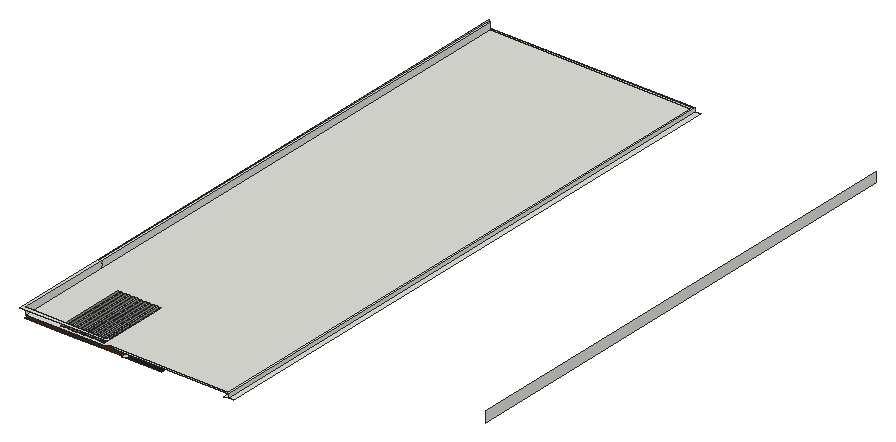
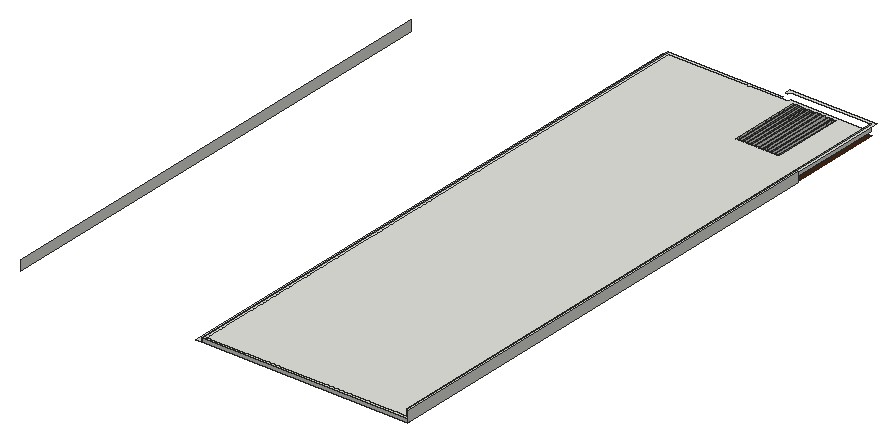
# SketchUp Ruby script. Lengths in inches.
U = 1.inch
M = Sketchup.active_model
def pt(a) = Geom::Point3d.new(a.map { |v| v * U })
def face(e, loops, mat)
  f = e.add_face(loops[0].map { |a| pt(a) })
  loops[1..].each { |l| e.add_face(l.map { |a| pt(a) }).erase! }
  f.material = f.back_material = mat if mat
  f
end
# faces: each face lists its corners as indices into pts; further lists are holes
def faces(e, pts, list, mat = nil) = list.each { |f| face(e, (f[0].is_a?(Array) ? f : [f]).map { |l| l.map { |i| pts[i] } }, mat) }
# xy, xz, yz: faces in a plane at the given z, y or x. An outline is a flat list of corners, or four numbers for a rectangle; further outlines are holes
def ring(l) = l.size == 4 ? [[l[0], l[1]], [l[2], l[1]], [l[2], l[3]], [l[0], l[3]]] : l.each_slice(2).to_a
def flat(e, list, mat, &to3) = list.each { |f| face(e, (f[0].is_a?(Array) ? f : [f]).map { |l| ring(l).map { |u, v| to3.(u, v) } }, mat) }
def xy(e, z, list, mat = nil) = flat(e, list, mat) { |x, y| [x, y, z] }
def xz(e, y, list, mat = nil) = flat(e, list, mat) { |x, z| [x, y, z] }
def yz(e, x, list, mat = nil) = flat(e, list, mat) { |y, z| [x, y, z] }
def lines(e, pts, list) = list.each { |a, b| e.add_line(pt(pts[a]), pt(pts[b])) }
# prism: a flat outline (further loops are holes) pulled along v
def prism(e, loops, v, mat = nil)
  f = face(e, loops, mat); d = Geom::Vector3d.new(v.map { |x| x * U })
  f.pushpull(f.normal.samedirection?(d) ? d.length : -d.length)
end
def box(e, o, s, mat = nil) = prism(e, [[o, [o[0] + s[0], o[1], o[2]], [o[0] + s[0], o[1] + s[1], o[2]], [o[0], o[1] + s[1], o[2]]]], [0, 0, s[2]], mat)
def at(x, y, z, deg = 0) = Geom::Transformation.translation(pt([x, y, z])) * Geom::Transformation.rotation(ORIGIN, Z_AXIS, deg.degrees)
def axes(o, x, y, z) = Geom::Transformation.new([*x, 0, *y, 0, *z, 0, *pt(o).to_a, 1])
def part(name) = M.definitions.add(name)
# library, detail: a bought-in or finely detailed component or shape, given as its bounding box
def library(name, o, s) = part(name).tap { |d| box(d.entities, o, s) }
def detail(e, o, s) = box(e.add_group.entities, o, s)
def put(e, d, t, mat = nil) = e.add_instance(d, t).tap { |i| i.material = mat if mat }
def group(e, t, mat = nil) = e.add_group.tap { |g| g.transformation = t; g.material = mat if mat }.entities
root = M.entities
M.materials.add("[Color M08]").color = [30, 30, 30]
M.materials.add("[Field Square Tile]").color = [211, 167, 108]
M.materials.add("[Granite Light Gray]").color = [149, 148, 144]
M.materials.add("[Wood Veneer 01]").color = [66, 38, 20]
xy(root,380.5,[[2434.04,511.08,2434.04,1825.82,1986.28,1825.82,1986.28,762.17,2202.28,762.17,2202.28,727.2,1976.47,727.2,1976.47,1835.625,2443.85,1835.625,2443.85,511.08],[2202.28,511.08,2211.2,589.83],[2443.85,511.08,2455.66,1835.625],[2202.28,589.83,2202.28,762.17,1986.28,762.17,1986.28,1825.82,2434.04,1825.82,2434.04,589.83,2387.27,589.83,2387.27,697.21,2291.96,697.21,2291.96,738.02,2211.2,738.02,2211.2,697.21,2202.58,697.21,2202.58,589.83],[2202.58,589.83,2211.2,697.21],
  [2291.96,589.83,2387.27,697.21],[2211.2,697.21,2291.96,738.02]])
xy(root,380.5,[[2211.2,511.08,2291.96,697.21]],"[Color M08]")
xy(root,380.5,[[[1981.3,512.27,2053.23,727.2],[1998.33,606.01,1999.85,606.38,2001.23,607.14,2002.36,608.22,2003.17,609.56,2003.6,611.0625,2003.64,612.63,2003.26,614.15,2002.51,615.52,2001.42,616.65,2000.08,617.46,1998.58,617.9,1997.01,617.93,1995.49,617.56,1994.12,616.81,1992.99,615.72,1992.18,614.38,1991.74,612.875,1991.71,611.3125,1992.08,609.79,1992.84,608.42,1993.92,607.29,1995.26,606.48,1996.77,606.04],[2038.08,606.01,2039.6,606.38,2040.98,607.14,2042.11,608.22,2042.92,609.56,2043.35,611.0625,2043.39,612.63,2043.01,614.15,2042.26,615.52,2041.17,616.65,2039.83,617.46,2038.33,617.9,2036.76,617.93,2035.24,617.56,2033.87,616.81,2032.74,615.72,2031.93,614.38,2031.49,612.875,2031.46,611.3125,2031.83,609.79,2032.59,608.42,2033.67,607.29,2035.01,606.48,2036.52,606.04],[1998.33,554.26,1999.85,554.63,2001.23,555.39,2002.36,556.47,2003.17,557.81,2003.6,559.3125,2003.64,560.88,2003.26,562.4,2002.51,563.77,2001.42,564.9,2000.08,565.71,1998.58,566.15,1997.01,566.18,1995.49,565.81,1994.12,565.06,1992.99,563.97,1992.18,562.63,1991.74,561.125,1991.71,559.5625,1992.08,558.04,1992.84,556.67,1993.92,555.54,1995.26,554.73,1996.77,554.29],[2038.08,554.26,2039.6,554.63,2040.98,555.39,2042.11,556.47,2042.92,557.81,2043.35,559.3125,2043.39,560.88,2043.01,562.4,2042.26,563.77,2041.17,564.9,2039.83,565.71,2038.33,566.15,2036.76,566.18,2035.24,565.81,2033.87,565.06,2032.74,563.97,2031.93,562.63,2031.49,561.125,2031.46,559.5625,2031.83,558.04,2032.59,556.67,2033.67,555.54,2035.01,554.73,2036.52,554.29],[1998.33,523.51,1999.85,523.88,2001.23,524.64,2002.36,525.72,2003.17,527.06,2003.6,528.5625,2003.64,530.13,2003.26,531.65,2002.51,533.02,2001.42,534.15,2000.08,534.96,1998.58,535.4,1997.01,535.43,1995.49,535.06,1994.12,534.31,1992.99,533.22,1992.18,531.88,1991.74,530.375,1991.71,528.8125,1992.08,527.29,1992.84,525.92,1993.92,524.79,1995.26,523.98,1996.77,523.54],[2038.08,523.51,2039.6,523.88,2040.98,524.64,2042.11,525.72,2042.92,527.06,2043.35,528.5625,2043.39,530.13,2043.01,531.65,2042.26,533.02,2041.17,534.15,2039.83,534.96,2038.33,535.4,2036.76,535.43,2035.24,535.06,2033.87,534.31,2032.74,533.22,2031.93,531.88,2031.49,530.375,2031.46,528.8125,2031.83,527.29,2032.59,525.92,2033.67,524.79,2035.01,523.98,2036.52,523.54],[1998.33,666.01,1999.85,666.38,2001.23,667.14,2002.36,668.22,2003.17,669.56,2003.6,671.0625,2003.64,672.63,2003.26,674.15,2002.51,675.52,2001.42,676.65,2000.08,677.46,1998.58,677.9,1997.01,677.93,1995.49,677.56,1994.12,676.81,1992.99,675.72,1992.18,674.38,1991.74,672.875,1991.71,671.3125,1992.08,669.79,1992.84,668.42,1993.92,667.29,1995.26,666.48,1996.77,666.04],[2038.08,666.01,2039.6,666.38,2040.98,667.14,2042.11,668.22,2042.92,669.56,2043.35,671.0625,2043.39,672.63,2043.01,674.15,2042.26,675.52,2041.17,676.65,2039.83,677.46,2038.33,677.9,2036.76,677.93,2035.24,677.56,2033.87,676.81,2032.74,675.72,2031.93,674.38,2031.49,672.875,2031.46,671.3125,2031.83,669.79,2032.59,668.42,2033.67,667.29,2035.01,666.48,2036.52,666.04]],[[2053.23,512.27,2202.28,727.2],[2148.68,519.43,2154.93,680.49],[2139.56,519.43,2145.81,680.49],[2130.43,519.43,2136.68,680.49],[2121.31,519.43,2127.56,680.49],[2112.18,519.43,2118.43,680.49],[2103.06,519.43,2109.31,680.49],[2093.93,519.43,2100.18,680.49],[2084.81,519.43,2091.06,680.49],[2075.68,519.43,2081.93,680.49],[2066.56,519.43,2072.81,680.49],[2057.43,519.43,2063.68,680.49]]],"[Wood Veneer 01]")
xy(root,381.875,[[1998.33,554.26,1996.77,554.29,1995.26,554.73,1993.92,555.54,1992.84,556.67,1992.08,558.04,1991.71,559.5625,1991.74,561.125,1992.18,562.63,1992.99,563.97,1994.12,565.06,1995.49,565.81,1997.01,566.18,1998.58,566.15,2000.08,565.71,2001.42,564.9,2002.51,563.77,2003.26,562.4,2003.64,560.88,2003.6,559.3125,2003.17,557.81,2002.36,556.47,2001.23,555.39,1999.85,554.63],[2038.08,554.26,2036.52,554.29,2035.01,554.73,2033.67,555.54,2032.59,556.67,2031.83,558.04,2031.46,559.5625,2031.49,561.125,2031.93,562.63,2032.74,563.97,2033.87,565.06,2035.24,565.81,2036.76,566.18,2038.33,566.15,2039.83,565.71,2041.17,564.9,2042.26,563.77,2043.01,562.4,2043.39,560.88,2043.35,559.3125,2042.92,557.81,2042.11,556.47,2040.98,555.39,2039.6,554.63],[1998.33,606.01,1996.77,606.04,1995.26,606.48,1993.92,607.29,1992.84,608.42,1992.08,609.79,1991.71,611.3125,1991.74,612.875,1992.18,614.38,1992.99,615.72,1994.12,616.81,1995.49,617.56,1997.01,617.93,1998.58,617.9,2000.08,617.46,2001.42,616.65,2002.51,615.52,2003.26,614.15,2003.64,612.63,2003.6,611.0625,2003.17,609.56,2002.36,608.22,2001.23,607.14,1999.85,606.38],[2038.08,606.01,2036.52,606.04,2035.01,606.48,2033.67,607.29,2032.59,608.42,2031.83,609.79,2031.46,611.3125,2031.49,612.875,2031.93,614.38,2032.74,615.72,2033.87,616.81,2035.24,617.56,2036.76,617.93,2038.33,617.9,2039.83,617.46,2041.17,616.65,2042.26,615.52,2043.01,614.15,2043.39,612.63,2043.35,611.0625,2042.92,609.56,2042.11,608.22,2040.98,607.14,2039.6,606.38],[1998.33,666.01,1996.77,666.04,1995.26,666.48,1993.92,667.29,1992.84,668.42,1992.08,669.79,1991.71,671.3125,1991.74,672.875,1992.18,674.38,1992.99,675.72,1994.12,676.81,1995.49,677.56,1997.01,677.93,1998.58,677.9,2000.08,677.46,2001.42,676.65,2002.51,675.52,2003.26,674.15,2003.64,672.63,2003.6,671.0625,2003.17,669.56,2002.36,668.22,2001.23,667.14,1999.85,666.38],
  [2038.08,666.01,2036.52,666.04,2035.01,666.48,2033.67,667.29,2032.59,668.42,2031.83,669.79,2031.46,671.3125,2031.49,672.875,2031.93,674.38,2032.74,675.72,2033.87,676.81,2035.24,677.56,2036.76,677.93,2038.33,677.9,2039.83,677.46,2041.17,676.65,2042.26,675.52,2043.01,674.15,2043.39,672.63,2043.35,671.0625,2042.92,669.56,2042.11,668.22,2040.98,667.14,2039.6,666.38]],"[Field Square Tile]")
xy(root,388.625,[[[1982.81,510.87,2166.13,510.87,2166.13,517.43,2437.5,517.43,2437.5,1829.28,1982.81,1829.28],[2057.43,519.43,2063.68,680.49],[2066.56,519.43,2072.81,680.49],[2075.68,519.43,2081.93,680.49],[2084.81,519.43,2091.06,680.49],[2093.93,519.43,2100.18,680.49],[2103.06,519.43,2109.31,680.49],[2112.18,519.43,2118.43,680.49],[2121.31,519.43,2127.56,680.49],[2130.43,519.43,2136.68,680.49],[2139.56,519.43,2145.81,680.49],[2148.68,519.43,2154.93,680.49]],[2183.1875,511.08,2443.85,511.08,2443.85,1835.625,1976.47,1835.625,1982.81,1829.28,2437.5,1829.28,2437.5,517.43,2183.1875,517.43]])
xy(root,403.8125,[[1976.47,504.52,2172.48,504.52,2172.48,517.43,2166.13,517.43,2166.13,510.87,1982.81,510.87,1982.81,1829.28,1976.47,1835.625]])
xz(root,680.49,[[2057.43,380.5,2063.68,388.625],[2066.56,380.5,2072.81,388.625],[2075.68,380.5,2081.93,388.625],[2084.81,380.5,2091.06,388.625],[2093.93,380.5,2100.18,388.625],
  [2103.06,380.5,2109.31,388.625],[2112.18,380.5,2118.43,388.625],[2121.31,380.5,2127.56,388.625],[2130.43,380.5,2136.68,388.625],[2139.56,380.5,2145.81,388.625],
  [2148.68,380.5,2154.93,388.625]],"[Granite Light Gray]")
xz(root,1835.625,[[1976.47,380.5,2443.85,388.625]])
yz(root,1976.47,[[727.2,380.5,1835.625,403.8125]])
yz(root,1982.81,[[510.87,388.625,727.2,403.8125],[727.2,388.625,1829.28,403.8125]])
yz(root,2057.43,[[519.43,380.5,680.49,388.625]],"[Granite Light Gray]")
yz(root,2063.68,[[519.43,380.5,680.49,388.625]])
yz(root,2066.56,[[519.43,380.5,680.49,388.625]],"[Granite Light Gray]")
yz(root,2072.81,[[519.43,380.5,680.49,388.625]])
yz(root,2075.68,[[519.43,380.5,680.49,388.625]],"[Granite Light Gray]")
yz(root,2081.93,[[519.43,380.5,680.49,388.625]])
yz(root,2084.81,[[519.43,380.5,680.49,388.625]],"[Granite Light Gray]")
yz(root,2091.06,[[519.43,380.5,680.49,388.625]])
yz(root,2093.93,[[519.43,380.5,680.49,388.625]],"[Granite Light Gray]")
yz(root,2100.18,[[519.43,380.5,680.49,388.625]])
yz(root,2103.06,[[519.43,380.5,680.49,388.625]],"[Granite Light Gray]")
yz(root,2109.31,[[519.43,380.5,680.49,388.625]])
yz(root,2112.18,[[519.43,380.5,680.49,388.625]],"[Granite Light Gray]")
yz(root,2118.43,[[519.43,380.5,680.49,388.625]])
yz(root,2121.31,[[519.43,380.5,680.49,388.625]],"[Granite Light Gray]")
yz(root,2127.56,[[519.43,380.5,680.49,388.625]])
yz(root,2130.43,[[519.43,380.5,680.49,388.625]],"[Granite Light Gray]")
yz(root,2136.68,[[519.43,380.5,680.49,388.625]])
yz(root,2139.56,[[519.43,380.5,680.49,388.625]],"[Granite Light Gray]")
yz(root,2145.81,[[519.43,380.5,680.49,388.625]])
yz(root,2148.68,[[519.43,380.5,680.49,388.625]],"[Granite Light Gray]")
yz(root,2154.93,[[519.43,380.5,680.49,388.625]])
yz(root,2443.85,[[511.08,380.5,1835.625,388.625]])
yz(root,2855.22,[[727.2,380.5,1835.625,403.8125]])
p = [[1996.77,554.29,380.5],[1995.26,554.73,380.5],[1995.26,554.73,381.875],[1996.77,554.29,381.875],[1998.33,554.26,380.5],[1998.33,554.26,381.875],
  [1999.85,554.63,380.5],[1999.85,554.63,381.875],[2036.52,554.29,380.5],[2035.01,554.73,380.5],[2035.01,554.73,381.875],[2036.52,554.29,381.875],
  [2038.08,554.26,380.5],[2038.08,554.26,381.875],[2039.6,554.63,380.5],[2039.6,554.63,381.875],[2001.23,555.39,380.5],[2001.23,555.39,381.875],
  [2040.98,555.39,380.5],[2040.98,555.39,381.875],[1993.92,555.54,380.5],[1993.92,555.54,381.875],[2033.67,555.54,380.5],[2033.67,555.54,381.875],
  [2002.36,556.47,380.5],[2002.36,556.47,381.875],[2042.11,556.47,380.5],[2042.11,556.47,381.875],[1992.84,556.67,380.5],[1992.84,556.67,381.875],
  [2032.59,556.67,380.5],[2032.59,556.67,381.875],[2003.17,557.81,380.5],[2003.17,557.81,381.875],[2042.92,557.81,380.5],[2042.92,557.81,381.875],
  [1992.08,558.04,380.5],[1992.08,558.04,381.875],[2031.83,558.04,380.5],[2031.83,558.04,381.875],[2003.6,559.3125,380.5],[2003.6,559.3125,381.875],
  [2043.35,559.3125,380.5],[2043.35,559.3125,381.875],[1991.71,559.5625,380.5],[1991.71,559.5625,381.875],[2031.46,559.5625,380.5],[2031.46,559.5625,381.875],
  [2003.64,560.88,380.5],[2003.64,560.88,381.875],[2043.39,560.88,380.5],[2043.39,560.88,381.875],[1991.74,561.125,380.5],[1991.74,561.125,381.875],
  [2031.49,561.125,380.5],[2031.49,561.125,381.875],[2003.26,562.4,380.5],[2003.26,562.4,381.875],[2043.01,562.4,380.5],[2043.01,562.4,381.875],
  [1992.18,562.63,380.5],[1992.18,562.63,381.875],[2031.93,562.63,380.5],[2031.93,562.63,381.875],[2002.51,563.77,380.5],[2002.51,563.77,381.875],
  [2042.26,563.77,380.5],[2042.26,563.77,381.875],[1992.99,563.97,380.5],[1992.99,563.97,381.875],[2032.74,563.97,380.5],[2032.74,563.97,381.875],
  [2001.42,564.9,380.5],[2001.42,564.9,381.875],[2041.17,564.9,380.5],[2041.17,564.9,381.875],[1994.12,565.06,380.5],[1994.12,565.06,381.875],
  [2033.87,565.06,380.5],[2033.87,565.06,381.875],[2000.08,565.71,380.5],[2000.08,565.71,381.875],[2039.83,565.71,380.5],[2039.83,565.71,381.875],
  [1995.49,565.81,380.5],[1995.49,565.81,381.875],[2035.24,565.81,380.5],[2035.24,565.81,381.875],[1998.58,566.15,380.5],[1998.58,566.15,381.875],
  [2038.33,566.15,380.5],[2038.33,566.15,381.875],[1997.01,566.18,380.5],[1997.01,566.18,381.875],[2036.76,566.18,380.5],[2036.76,566.18,381.875],
  [1996.77,606.04,380.5],[1995.26,606.48,380.5],[1995.26,606.48,381.875],[1996.77,606.04,381.875],[1998.33,606.01,380.5],[1998.33,606.01,381.875],
  [1999.85,606.38,380.5],[1999.85,606.38,381.875],[2036.52,606.04,380.5],[2035.01,606.48,380.5],[2035.01,606.48,381.875],[2036.52,606.04,381.875],
  [2038.08,606.01,380.5],[2038.08,606.01,381.875],[2039.6,606.38,380.5],[2039.6,606.38,381.875],[2001.23,607.14,380.5],[2001.23,607.14,381.875],
  [2040.98,607.14,380.5],[2040.98,607.14,381.875],[1993.92,607.29,380.5],[1993.92,607.29,381.875],[2033.67,607.29,380.5],[2033.67,607.29,381.875],
  [2002.36,608.22,380.5],[2002.36,608.22,381.875],[2042.11,608.22,380.5],[2042.11,608.22,381.875],[1992.84,608.42,380.5],[1992.84,608.42,381.875],
  [2032.59,608.42,380.5],[2032.59,608.42,381.875],[2003.17,609.56,380.5],[2003.17,609.56,381.875],[2042.92,609.56,380.5],[2042.92,609.56,381.875],
  [1992.08,609.79,380.5],[1992.08,609.79,381.875],[2031.83,609.79,380.5],[2031.83,609.79,381.875],[2003.6,611.0625,380.5],[2003.6,611.0625,381.875],
  [2043.35,611.0625,380.5],[2043.35,611.0625,381.875],[1991.71,611.3125,380.5],[1991.71,611.3125,381.875],[2031.46,611.3125,380.5],[2031.46,611.3125,381.875],
  [2003.64,612.63,380.5],[2003.64,612.63,381.875],[2043.39,612.63,380.5],[2043.39,612.63,381.875],[1991.74,612.875,380.5],[1991.74,612.875,381.875],
  [2031.49,612.875,380.5],[2031.49,612.875,381.875],[2003.26,614.15,380.5],[2003.26,614.15,381.875],[2043.01,614.15,380.5],[2043.01,614.15,381.875],
  [1992.18,614.38,380.5],[1992.18,614.38,381.875],[2031.93,614.38,380.5],[2031.93,614.38,381.875],[2002.51,615.52,380.5],[2002.51,615.52,381.875],
  [2042.26,615.52,380.5],[2042.26,615.52,381.875],[1992.99,615.72,380.5],[1992.99,615.72,381.875],[2032.74,615.72,380.5],[2032.74,615.72,381.875],
  [2001.42,616.65,380.5],[2001.42,616.65,381.875],[2041.17,616.65,380.5],[2041.17,616.65,381.875],[1994.12,616.81,380.5],[1994.12,616.81,381.875],
  [2033.87,616.81,380.5],[2033.87,616.81,381.875],[2000.08,617.46,380.5],[2000.08,617.46,381.875],[2039.83,617.46,380.5],[2039.83,617.46,381.875],
  [1995.49,617.56,380.5],[1995.49,617.56,381.875],[2035.24,617.56,380.5],[2035.24,617.56,381.875],[1998.58,617.9,380.5],[1998.58,617.9,381.875],
  [2038.33,617.9,380.5],[2038.33,617.9,381.875],[1997.01,617.93,380.5],[1997.01,617.93,381.875],[2036.76,617.93,380.5],[2036.76,617.93,381.875],
  [1996.77,666.04,380.5],[1995.26,666.48,380.5],[1995.26,666.48,381.875],[1996.77,666.04,381.875],[1998.33,666.01,380.5],[1998.33,666.01,381.875],
  [1999.85,666.38,380.5],[1999.85,666.38,381.875],[2036.52,666.04,380.5],[2035.01,666.48,380.5],[2035.01,666.48,381.875],[2036.52,666.04,381.875],
  [2038.08,666.01,380.5],[2038.08,666.01,381.875],[2039.6,666.38,380.5],[2039.6,666.38,381.875],[2001.23,667.14,380.5],[2001.23,667.14,381.875],
  [2040.98,667.14,380.5],[2040.98,667.14,381.875],[1993.92,667.29,380.5],[1993.92,667.29,381.875],[2033.67,667.29,380.5],[2033.67,667.29,381.875],
  [2002.36,668.22,380.5],[2002.36,668.22,381.875],[2042.11,668.22,380.5],[2042.11,668.22,381.875],[1992.84,668.42,380.5],[1992.84,668.42,381.875],
  [2032.59,668.42,380.5],[2032.59,668.42,381.875],[2003.17,669.56,380.5],[2003.17,669.56,381.875],[2042.92,669.56,380.5],[2042.92,669.56,381.875],
  [1992.08,669.79,380.5],[1992.08,669.79,381.875],[2031.83,669.79,380.5],[2031.83,669.79,381.875],[2003.6,671.0625,380.5],[2003.6,671.0625,381.875],
  [2043.35,671.0625,380.5],[2043.35,671.0625,381.875],[1991.71,671.3125,380.5],[1991.71,671.3125,381.875],[2031.46,671.3125,380.5],[2031.46,671.3125,381.875],
  [2003.64,672.63,380.5],[2003.64,672.63,381.875],[2043.39,672.63,380.5],[2043.39,672.63,381.875],[1991.74,672.875,380.5],[1991.74,672.875,381.875],
  [2031.49,672.875,380.5],[2031.49,672.875,381.875],[2003.26,674.15,380.5],[2003.26,674.15,381.875],[2043.01,674.15,380.5],[2043.01,674.15,381.875],
  [1992.18,674.38,380.5],[1992.18,674.38,381.875],[2031.93,674.38,380.5],[2031.93,674.38,381.875],[2002.51,675.52,380.5],[2002.51,675.52,381.875],
  [2042.26,675.52,380.5],[2042.26,675.52,381.875],[1992.99,675.72,380.5],[1992.99,675.72,381.875],[2032.74,675.72,380.5],[2032.74,675.72,381.875],
  [2001.42,676.65,380.5],[2001.42,676.65,381.875],[2041.17,676.65,380.5],[2041.17,676.65,381.875],[1994.12,676.81,380.5],[1994.12,676.81,381.875],
  [2033.87,676.81,380.5],[2033.87,676.81,381.875],[2000.08,677.46,380.5],[2000.08,677.46,381.875],[2039.83,677.46,380.5],[2039.83,677.46,381.875],
  [1995.49,677.56,380.5],[1995.49,677.56,381.875],[2035.24,677.56,380.5],[2035.24,677.56,381.875],[1998.58,677.9,380.5],[1998.58,677.9,381.875],
  [2038.33,677.9,380.5],[2038.33,677.9,381.875],[1997.01,677.93,380.5],[1997.01,677.93,381.875],[2036.76,677.93,380.5],[2036.76,677.93,381.875],
  [1982.81,1829.28,388.625],[1976.47,1835.625,388.625],[1976.47,1835.625,403.8125],[1982.81,1829.28,403.8125]]
faces(root,p,[[0,1,2,3],[4,0,3,5],[6,4,5,7],[8,9,10,11],[12,8,11,13],[14,12,13,15],[16,6,7,17],[18,14,15,19],
  [1,20,21,2],[9,22,23,10],[24,16,17,25],[26,18,19,27],[20,28,29,21],[22,30,31,23],[32,24,25,33],[34,26,27,35],
  [28,36,37,29],[30,38,39,31],[40,32,33,41],[42,34,35,43],[36,44,45,37],[38,46,47,39],[48,40,41,49],[50,42,43,51],
  [44,52,53,45],[46,54,55,47],[56,48,49,57],[58,50,51,59],[52,60,61,53],[54,62,63,55],[64,56,57,65],[66,58,59,67],
  [60,68,69,61],[62,70,71,63],[72,64,65,73],[74,66,67,75],[68,76,77,69],[70,78,79,71],[80,72,73,81],[82,74,75,83],
  [76,84,85,77],[78,86,87,79],[88,80,81,89],[90,82,83,91],[84,92,93,85],[86,94,95,87],[92,88,89,93],[94,90,91,95],
  [96,97,98,99],[100,96,99,101],[102,100,101,103],[104,105,106,107],[108,104,107,109],[110,108,109,111],[112,102,103,113],[114,110,111,115],
  [97,116,117,98],[105,118,119,106],[120,112,113,121],[122,114,115,123],[116,124,125,117],[118,126,127,119],[128,120,121,129],[130,122,123,131],
  [124,132,133,125],[126,134,135,127],[136,128,129,137],[138,130,131,139],[132,140,141,133],[134,142,143,135],[144,136,137,145],[146,138,139,147],
  [140,148,149,141],[142,150,151,143],[152,144,145,153],[154,146,147,155],[148,156,157,149],[150,158,159,151],[160,152,153,161],[162,154,155,163],
  [156,164,165,157],[158,166,167,159],[168,160,161,169],[170,162,163,171],[164,172,173,165],[166,174,175,167],[176,168,169,177],[178,170,171,179],
  [172,180,181,173],[174,182,183,175],[184,176,177,185],[186,178,179,187],[180,188,189,181],[182,190,191,183],[188,184,185,189],[190,186,187,191],
  [192,193,194,195],[196,192,195,197],[198,196,197,199],[200,201,202,203],[204,200,203,205],[206,204,205,207],[208,198,199,209],[210,206,207,211],
  [193,212,213,194],[201,214,215,202],[216,208,209,217],[218,210,211,219],[212,220,221,213],[214,222,223,215],[224,216,217,225],[226,218,219,227],
  [220,228,229,221],[222,230,231,223],[232,224,225,233],[234,226,227,235],[228,236,237,229],[230,238,239,231],[240,232,233,241],[242,234,235,243],
  [236,244,245,237],[238,246,247,239],[248,240,241,249],[250,242,243,251],[244,252,253,245],[246,254,255,247],[256,248,249,257],[258,250,251,259],
  [252,260,261,253],[254,262,263,255],[264,256,257,265],[266,258,259,267],[260,268,269,261],[262,270,271,263],[272,264,265,273],[274,266,267,275],
  [268,276,277,269],[270,278,279,271],[280,272,273,281],[282,274,275,283],[276,284,285,277],[278,286,287,279],[284,280,281,285],[286,282,283,287]],"[Field Square Tile]")
faces(root,p,[[288,289,290,291]])
